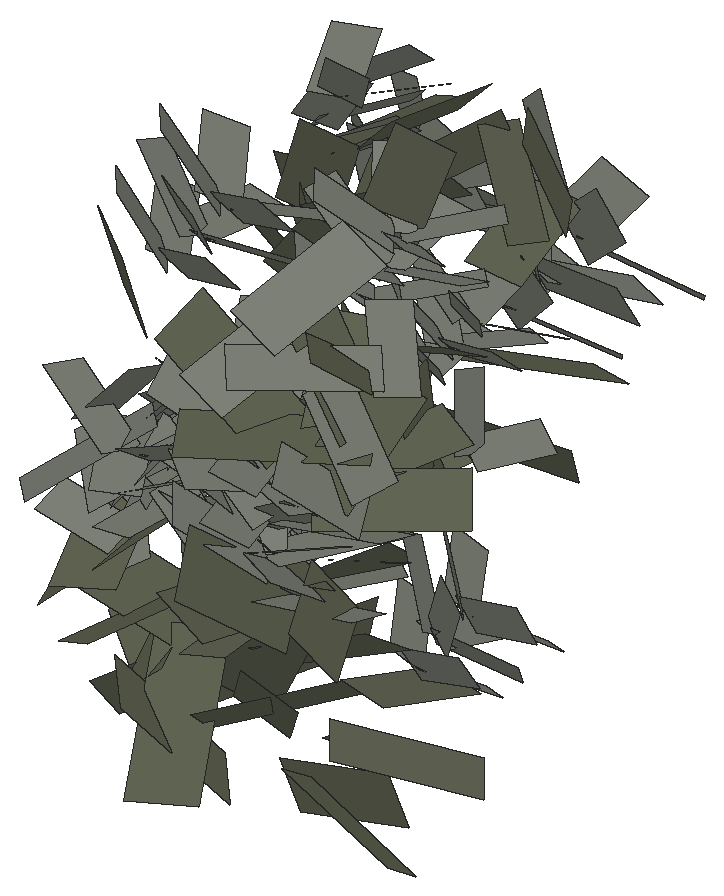
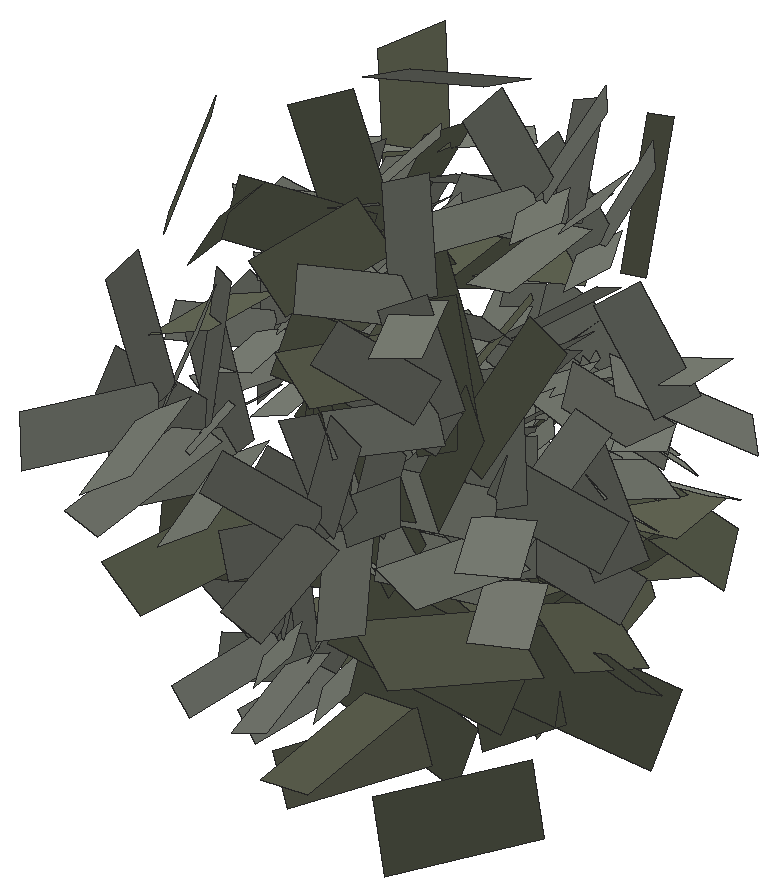
# SketchUp Ruby script. Lengths in inches.
U = 1.inch
M = Sketchup.active_model
def pt(a) = Geom::Point3d.new(a.map { |v| v * U })
def face(e, loops, mat)
  f = e.add_face(loops[0].map { |a| pt(a) })
  loops[1..].each { |l| e.add_face(l.map { |a| pt(a) }).erase! }
  f.material = f.back_material = mat if mat
  f
end
# faces: each face lists its corners as indices into pts; further lists are holes
def faces(e, pts, list, mat = nil) = list.each { |f| face(e, (f[0].is_a?(Array) ? f : [f]).map { |l| l.map { |i| pts[i] } }, mat) }
# xy, xz, yz: faces in a plane at the given z, y or x. An outline is a flat list of corners, or four numbers for a rectangle; further outlines are holes
def ring(l) = l.size == 4 ? [[l[0], l[1]], [l[2], l[1]], [l[2], l[3]], [l[0], l[3]]] : l.each_slice(2).to_a
def flat(e, list, mat, &to3) = list.each { |f| face(e, (f[0].is_a?(Array) ? f : [f]).map { |l| ring(l).map { |u, v| to3.(u, v) } }, mat) }
def xy(e, z, list, mat = nil) = flat(e, list, mat) { |x, y| [x, y, z] }
def xz(e, y, list, mat = nil) = flat(e, list, mat) { |x, z| [x, y, z] }
def yz(e, x, list, mat = nil) = flat(e, list, mat) { |y, z| [x, y, z] }
def lines(e, pts, list) = list.each { |a, b| e.add_line(pt(pts[a]), pt(pts[b])) }
# prism: a flat outline (further loops are holes) pulled along v
def prism(e, loops, v, mat = nil)
  f = face(e, loops, mat); d = Geom::Vector3d.new(v.map { |x| x * U })
  f.pushpull(f.normal.samedirection?(d) ? d.length : -d.length)
end
def box(e, o, s, mat = nil) = prism(e, [[o, [o[0] + s[0], o[1], o[2]], [o[0] + s[0], o[1] + s[1], o[2]], [o[0], o[1] + s[1], o[2]]]], [0, 0, s[2]], mat)
def at(x, y, z, deg = 0) = Geom::Transformation.translation(pt([x, y, z])) * Geom::Transformation.rotation(ORIGIN, Z_AXIS, deg.degrees)
def axes(o, x, y, z) = Geom::Transformation.new([*x, 0, *y, 0, *z, 0, *pt(o).to_a, 1])
def part(name) = M.definitions.add(name)
# library, detail: a bought-in or finely detailed component or shape, given as its bounding box
def library(name, o, s) = part(name).tap { |d| box(d.entities, o, s) }
def detail(e, o, s) = box(e.add_group.entities, o, s)
def put(e, d, t, mat = nil) = e.add_instance(d, t).tap { |i| i.material = mat if mat }
def group(e, t, mat = nil) = e.add_group.tap { |g| g.transformation = t; g.material = mat if mat }.entities
root = M.entities
M.materials.add("viburnumblaasdfas0df1w06d").color = [98, 102, 84]
M.materials.add("viburnumbladsadfasdfad0w122").color = [125, 129, 119]
c1 = part("Component\#315")
p = [[0.25,0,0],[2.05,0.01,0.35],[1.81,4.2,1.66],[0,4.19,1.3125]]
faces(c1.entities,p,[[0,1,2,3]],"viburnumbladsadfasdfad0w122")
c2 = part("viburnumblad2")
put(c2.entities,c1,axes([-19.23,-4.49,-32.18],[83.35428,0,0],[0,79.38502,0],[0,0,83.35428]))
c3 = part("Component\#314")
p = [[0.14,0,0],[2.58,0.05,0.25],[2.44,5.11,2.64],[0,5.05,2.39]]
faces(c3.entities,p,[[0,1,2,3]],"viburnumblaasdfas0df1w06d")
c4 = part("viburnumblad1\#2")
put(c4.entities,c3,axes([-37.25,6.23,19.31],[75.98784,0,0],[0,65.50676,0],[0,0,75.98784]))
put(root,c2,axes([1226.95,207.14,17.86],[0.01077,-0.01075,-0.00083],[0.01118,0.01095,0.00335],[-0.00168,-0.00283,0.01488]))
put(root,c4,axes([1239.8125,210.73,25.15],[-0.01089,-0.0066,0.00527],[0.00777,-0.0139,-0.00135],[0.00514,0.00164,0.01268]))
put(root,c2,axes([1231.69,209.11,19.34],[-0.00239,-0.01136,0.0048],[0.01232,-0.002,0.0014],[-0.0005,0.00498,0.01153]))
put(root,c2,axes([1236.75,207.28,26.68],[0.00842,-0.01125,-0.00685],[0.01063,0.01127,-0.00543],[0.00843,-0.00165,0.01307]))
put(root,c4,axes([1238.97,211.42,14.45],[-0.00936,-0.00465,0.0096],[0.00338,-0.01554,-0.00424],[0.01026,-0.00044,0.00979]))
put(root,c2,axes([1241.4,209.16,19.2],[-0.00545,0.00916,0.00529],[-0.00808,-0.00821,0.00589],[0.00818,-0.00089,0.00998]))
put(root,c4,axes([1236.82,210.48,12.36],[-0.00461,0.01011,0.01059],[-0.01024,-0.0125,0.00748],[0.01168,-0.00415,0.00905]))
put(root,c2,axes([1230.61,207.5,15.64],[0.00178,0.0105,0.00298],[-0.0098,0.00211,-0.00159],[-0.00226,-0.0026,0.01051]))
put(root,c4,axes([1230.86,209.27,23.78],[-0.01166,0.00571,0.00452],[-0.00151,-0.01177,0.01017],[0.0071,0.00732,0.00793]))
put(root,c2,axes([1237.0625,209.16,16.01],[-0.00958,0.01044,0.00206],[-0.00856,-0.00879,0.00474],[0.00514,0.00211,0.0132]))
put(root,c4,axes([1233.03,206.34,5.98],[0.01503,0.00487,0.00033],[-0.00521,0.01551,0.00826],[0.00191,-0.00687,0.0141]))
put(root,c2,axes([1236.97,210.84,15.95],[-0.00988,-0.00976,0.00351],[0.01049,-0.01076,-0.00039],[0.00277,0.00219,0.01388]))
put(root,c2,axes([1230.9,207.19,20.19],[0.00239,0.01136,-0.0048],[-0.01208,0.00314,0.00143],[0.00249,0.00434,0.01152]))
put(root,c2,axes([1236.56,210.93,20.37],[-0.01175,-0.00377,0.00233],[0.00341,-0.01191,-0.00208],[0.00284,-0.00132,0.01217]))
put(root,c4,axes([1229.6,206.2,11.54],[0.01155,-0.00606,0.00446],[0.00831,0.01316,-0.00362],[-0.00229,0.00493,0.01266]))
put(root,c4,axes([1233.6,207.74,21.8],[0.00835,-0.01477,-0.00252],[0.01522,0.00998,-0.00805],[0.00724,0.00145,0.01548]))
put(root,c4,axes([1234.6,209.79,5.19],[-0.01033,0.0106,0.00208],[-0.0106,-0.01173,0.00714],[0.00578,0.00298,0.01347]))
put(root,c4,axes([1227.57,208.05,12.29],[0.0081,-0.01447,0.00211],[0.01627,0.00971,0.00411],[-0.00412,0.00005,0.0162]))
put(root,c4,axes([1229.8,205.78,14.06],[0.01294,0.00473,-0.00003],[-0.00539,0.01473,-0.00308],[-0.00088,0.0025,0.01352]))
put(root,c2,axes([1230.54,208.45,17.9375],[0.007,-0.00987,0.00339],[0.00957,0.00618,-0.0018],[-0.00027,0.0039,0.01194]))
put(root,c2,axes([1235.37,206.35,25.32],[0.01184,-0.00027,-0.00922],[0.00172,0.01671,0.00172],[0.00948,-0.00223,0.01224]))
put(root,c2,axes([1237.53,206.63,28.62],[0.01234,-0.00028,-0.00961],[0.00159,0.01547,0.00159],[0.00948,-0.00223,0.01224]))
put(root,c4,axes([1234.72,212.03,12.13],[-0.01223,0.00026,0.00635],[-0.0009,-0.01592,-0.0011],[0.0063,-0.0012,0.0122]))
put(root,c4,axes([1237.41,209.01,20.64],[0.00084,0.01421,0.00442],[-0.01582,-0.0012,0.00687],[0.00595,-0.00438,0.01294]))
put(root,c2,axes([1229.92,209.05,17.31],[0.00604,-0.00926,0.00001],[0.00806,0.00526,0.00544],[-0.00456,-0.00296,0.00963]))
put(root,c2,axes([1228.79,210.32,19.83],[-0.00259,-0.01229,0.00001],[0.0107,-0.00225,0.00618],[-0.00604,0.00128,0.01094]))
put(root,c2,axes([1230.2,207.53,16.75],[0.01283,-0.0027,-0.00001],[0.00224,0.01066,-0.00301],[0.0007,0.00327,0.01211]))
put(root,c2,axes([1236.01,210.61,18.7],[-0.01046,0.00558,0.00416],[-0.00525,-0.01025,0.00054],[0.00396,-0.00141,0.01184]))
put(root,c2,axes([1235.65,211.38,17.42],[-0.01227,-0.00394,0.00243],[0.00307,-0.01072,-0.00188],[0.00284,-0.00132,0.01217]))
put(root,c2,axes([1235.74,210.03,17.37],[-0.00945,0.00658,-0.00199],[-0.00667,-0.00798,0.00533],[0.00164,0.00544,0.01021]))
put(root,c2,axes([1230.37,207.1,18.52],[0.01038,0.0062,-0.0034],[-0.00717,0.01088,-0.00204],[0.00185,0.00346,0.01194]))
put(root,c2,axes([1241.5,208.6,20.85],[0.00288,0.01252,0.00147],[-0.00904,0.00098,0.00938],[0.00888,-0.00309,0.00888]))
put(root,c2,axes([1229.48,207.8,16.87],[0.00856,0.00558,0.00422],[-0.00642,0.00891,0.00123],[-0.00278,-0.00341,0.01014]))
put(root,c4,axes([1237.26,210.58,6.97],[0.00066,-0.01186,0.00699],[0.01121,-0.00532,-0.01007],[0.0098,0.00532,0.0081]))
put(root,c2,axes([1236.1,211.13,18.5],[-0.01151,-0.00142,0.00146],[0.00195,-0.0101,0.00555],[0.00059,0.0057,0.01018]))
put(root,c2,axes([1235.61,208.65,14.84],[-0.00037,0.01298,-0.00224],[-0.01317,0.00059,0.00559],[0.0056,0.0024,0.01296]))
put(root,c2,axes([1235.57,209.6875,20.35],[-0.00304,0.01166,0.00355],[-0.01127,-0.00408,0.00376],[0.00464,-0.00228,0.01145]))
put(root,c4,axes([1234.08,208.98,8.375],[0.00317,-0.01127,0.00742],[0.01555,0.00409,-0.00043],[-0.00159,0.00725,0.0117]))
put(root,c2,axes([1230.28,208.26,14.39],[0.0081,0.00545,0.00286],[-0.00642,0.00891,0.00123],[-0.00184,-0.00279,0.01054]))
put(root,c4,axes([1240.42,209.32,22.41],[0.00107,0.01287,0.00071],[-0.01171,0.00034,0.00907],[0.0079,-0.00141,0.00892]))
put(root,c2,axes([1235.64,210.98,14.51],[-0.0002,-0.01371,0.00098],[0.01527,-0.0004,-0.00242],[0.00226,0.00098,0.01411]))
put(root,c4,axes([1235.23,211.95,7.27],[-0.01191,-0.00399,0.00577],[0.00688,-0.0137,0.00471],[0.00376,0.00597,0.01189]))
put(root,c2,axes([1235.0625,209.35,16.13],[-0.00179,0.01029,-0.00409],[-0.01223,-0.00094,0.00298],[0.00221,0.00457,0.01052]))
put(root,c2,axes([1235.72,211.41,16.8],[-0.00682,-0.00858,0.00405],[0.00958,-0.00605,0.00332],[-0.00034,0.0052,0.01046]))
put(root,c2,axes([1236.49,209,18.14],[0.00021,0.01428,-0.00102],[-0.01317,0.00059,0.00559],[0.00561,0.00086,0.01315]))
put(root,c4,axes([1238.84,208.55,20.49],[0.01029,0.00428,-0.00658],[0.00078,0.01194,0.00879],[0.00737,-0.00649,0.00685]))
put(root,c2,axes([1235.54,211.9375,19.16],[-0.00616,-0.01091,-0.00086],[0.01132,-0.00616,-0.00282],[0.00193,-0.00206,0.01224]))
put(root,c2,axes([1229.75,208.8,15.67],[0.01032,-0.0026,0.00299],[0.00135,0.01024,0.00424],[-0.00373,-0.00356,0.00978]))
put(root,c4,axes([1233.08,211.32,9.65],[-0.00358,0.0126,0.00711],[-0.01496,-0.00708,0.005],[0.00656,-0.00511,0.01237]))
put(root,c4,axes([1234.71,212.67,14.61],[-0.00859,-0.01039,0.00287],[0.01161,-0.0105,-0.00325],[0.004,0.00034,0.01318]))
put(root,c2,axes([1234.88,210.27,17.48],[-0.00324,0.01089,0.00211],[-0.01127,-0.00408,0.00376],[0.00428,-0.00101,0.01177]))
put(root,c2,axes([1231.44,211.86,25.56],[-0.00734,-0.00647,0.00686],[0.01022,-0.00834,0.00267],[0.00284,0.00722,0.00872]))
put(root,c2,axes([1230.25,208.55,19.69],[0.01229,-0.00259,-0.00001],[0.00249,0.01185,-0.00335],[0.0007,0.00327,0.01211]))
put(root,c2,axes([1231.46,210.52,26.4],[-0.00945,0.00892,-0.00145],[-0.0064,-0.00533,0.00736],[0.00487,0.007,0.00802]))
put(root,c2,axes([1236.94,211.5,17.84],[-0.00021,-0.01428,0.00102],[0.01414,-0.00037,-0.00224],[0.00226,0.00098,0.01411]))
put(root,c2,axes([1232.37,211.98,26.84],[-0.01181,0.00128,0.00407],[0.00154,-0.01046,0.00743],[0.00382,0.0075,0.00815]))
put(root,c2,axes([1228.44,210.26,17.97],[0.0062,-0.01038,0.0034],[0.00931,0.00714,0.00482],[-0.00586,0.00014,0.01111]))
put(root,c2,axes([1234.8,211.15,15.55],[0.00176,-0.01022,0.00282],[0.01152,0.00195,-0.00013],[-0.00039,0.00304,0.01127]))
put(root,c2,axes([1235.05,210.2,18.96],[-0.00186,0.01072,-0.00426],[-0.01132,-0.00087,0.00276],[0.00221,0.00457,0.01052]))
put(root,c4,axes([1232.05,209.32,7.57],[0.00865,0.00658,0.00734],[-0.00992,0.01145,0.00143],[-0.0049,-0.0056,0.0108]))
put(root,c2,axes([1228.44,209.39,16.52],[0.01089,-0.00213,0.00325],[0.002,0.01232,0.0014],[-0.00372,-0.00076,0.01198]))
put(root,c4,axes([1233.8,208.63,13.37],[0.00989,0.00806,-0.00127],[-0.00946,0.01134,-0.00169],[0.00005,0.00193,0.01267]))
put(root,c2,axes([1235.39,211.86,20.9],[0.00304,-0.01166,-0.00355],[0.01206,0.00341,-0.00087],[0.00178,-0.0032,0.01202]))
put(root,c2,axes([1234.36,210.07,19.07],[0.00616,0.01091,0.00086],[-0.01009,0.00525,0.00563],[0.00448,-0.00342,0.01123]))
put(root,c2,axes([1241.47,209.95,24.9],[0.0051,0.01038,-0.00415],[-0.00729,0.00572,0.00502],[0.00694,0.00038,0.0084]))
put(root,c2,axes([1235.13,209.24,16.61],[0.00988,0.00976,-0.00351],[-0.00912,0.01058,0.00376],[0.00511,-0.00035,0.01338]))
put(root,c4,axes([1230.71,208.82,8.77],[0.01224,-0.00166,0.00834],[0.00122,0.01717,0.00163],[-0.00844,-0.00056,0.01227]))
put(root,c4,axes([1237.57,210.72,19.44],[0.00626,-0.00918,-0.00848],[0.01094,0.01129,-0.00412],[0.00772,-0.00395,0.00939]))
put(root,c2,axes([1235.2,212.26,12.91],[-0.0083,0.00785,-0.00197],[-0.00857,-0.00783,0.00492],[0.002,0.00498,0.01141]))
put(root,c4,axes([1233.21,208.9375,11.08],[0.01241,-0.00186,0.00262],[0.00291,0.01409,-0.00376],[-0.00201,0.00365,0.01212]))
put(root,c4,axes([1238.27,210.68,9.32],[0.00753,-0.01126,-0.00255],[0.00884,0.00827,-0.01044],[0.00867,0.00351,0.01012]))
put(root,c2,axes([1235.36,213.53,12.46],[-0.00925,-0.00862,0.00362],[0.00803,-0.00772,0.00213],[0.00081,0.00412,0.01188]))
put(root,c2,axes([1234.42,209.96,17.47],[0.00682,0.00858,-0.00405],[-0.00975,0.00742,-0.00069],[0.00196,0.0036,0.01094]))
put(root,c4,axes([1238.36,209.56,21.39],[0.00971,0.0077,-0.00377],[-0.00736,0.01191,0.00523],[0.00557,-0.00177,0.01033]))
put(root,c4,axes([1228.48,210.5625,6.375],[0.00095,-0.01143,0.01095],[0.01752,0.00456,0.00324],[-0.00472,0.01026,0.01113]))
put(root,c2,axes([1235.07,212.13,18.16],[0.00186,-0.01072,0.00426],[0.01152,0.00195,-0.00013],[-0.00059,0.00423,0.01088]))
put(root,c2,axes([1232.67,212.05,28.52],[-0.00905,0.00854,-0.00139],[-0.00711,-0.00593,0.00818],[0.00487,0.007,0.00802]))
put(root,c2,axes([1235.43,211.04,16.41],[0.00958,-0.01044,-0.00206],[0.01029,0.0098,-0.00181],[0.00273,-0.00027,0.01406]))
put(root,c2,axes([1235.79,213.48,13.95],[-0.01246,0.00054,0.00182],[0.00014,-0.01079,0.00417],[0.00189,0.00451,0.01162]))
put(root,c2,axes([1232.8,213.37,27.68],[-0.00765,-0.00673,0.00714],[0.00947,-0.00772,0.00247],[0.00284,0.00722,0.00872]))
put(root,c2,axes([1234.38,212.22,17.92],[0.00292,-0.01119,-0.00341],[0.01302,0.00368,-0.00094],[0.00178,-0.0032,0.01202]))
put(root,c4,axes([1232.87,213.8125,6.53],[-0.01405,-0.00766,0.00571],[0.01107,-0.01374,0.00878],[0.00057,0.00947,0.0141]))
put(root,c2,axes([1233.9375,210.29,15.875],[0.01201,0.00148,-0.00152],[-0.00157,0.01006,-0.00263],[0.00104,0.00309,0.01122]))
put(root,c2,axes([1234.1,211.2,16.97],[0.00945,-0.00658,0.00199],[0.00631,0.00831,-0.00248],[-0.00002,0.00335,0.01119]))
put(root,c2,axes([1231.55,211.11,27.68],[-0.00099,0.0108,-0.00603],[-0.01031,0.00186,0.00471],[0.00538,0.00602,0.00839]))
put(root,c4,axes([1235.24,212.59,4.09],[-0.00376,-0.0039,0.01194],[0.01323,-0.00731,0.00178],[0.00528,0.01082,0.0052]))
put(root,c4,axes([1236.1,213.6,18.02],[-0.00832,0.00937,0.00389],[-0.0091,-0.01059,0.00604],[0.00643,0.00098,0.01139]))
put(root,c2,axes([1231.43,213.02,26.63],[0.00099,-0.0108,0.00603],[0.0122,-0.00051,-0.00294],[0.0025,0.00634,0.00938]))
put(root,c2,axes([1235.53,213.02,15.8125],[-0.00876,0.00902,-0.0009],[-0.00857,-0.00783,0.00492],[0.00296,0.00403,0.01157]))
put(root,c2,axes([1234.4,210.62,20.88],[0.01175,0.00377,-0.00233],[-0.00262,0.01124,0.00497],[0.00358,-0.00416,0.0113]))
put(root,c4,axes([1234.46,213.24,9.36],[-0.00313,-0.01186,0.00638],[0.01559,-0.00367,0.00082],[0.00085,0.00636,0.01225]))
put(root,c2,axes([1235.8125,214.53,15.39],[-0.00886,-0.00826,0.00347],[0.00892,-0.00858,0.00237],[0.00081,0.00412,0.01188]))
put(root,c2,axes([1235.51,210.51,18.32],[0.01376,-0.00048,-0.00394],[0.00069,0.01429,0.00066],[0.00391,-0.00082,0.01375]))
put(root,c2,axes([1234.2,211.62,19.48],[0.01046,-0.00558,-0.00416],[0.00651,0.0105,0.0023],[0.00246,-0.00407,0.01163]))
put(root,c2,axes([1230.21,210.85,26.82],[0.00649,0.00565,-0.00743],[-0.0085,0.00924,-0.00029],[0.00584,0.00584,0.00823]))
put(root,c4,axes([1236.96,210.8125,19.46],[0.01206,-0.00628,-0.00336],[0.00668,0.01448,-0.00311],[0.00388,0.00091,0.01211]))
put(root,c2,axes([1234.02,211.2,18.62],[0.01151,0.00142,-0.00146],[-0.00175,0.01118,-0.00292],[0.00104,0.00309,0.01122]))
put(root,c4,axes([1236.94,215.24,19.97],[-0.01002,-0.00367,0.00577],[0.0058,-0.01266,0.00203],[0.00466,0.00382,0.01053]))
put(root,c2,axes([1234.54,212.33,14.47],[0.00007,0.01222,-0.00309],[-0.01226,0.00091,0.00331],[0.0034,0.00296,0.01177]))
put(root,c2,axes([1228.05,214.8,15.65],[-0.00906,-0.00899,0.00397],[0.00943,-0.00624,0.00738],[-0.00308,0.00772,0.01046]))
put(root,c2,axes([1234.68,214.47,13.89],[-0.00007,-0.01222,0.00309],[0.01323,-0.00017,-0.00035],[0.00036,0.00309,0.01221]))
put(root,c2,axes([1227.36,214.29,14.07],[0.00073,-0.01105,0.00534],[0.01289,0.00219,0.00278],[-0.00345,0.00543,0.01171]))
put(root,c2,axes([1230.29,212.33,27.51],[0.01181,-0.00128,-0.00407],[-0.00051,0.0116,-0.00495],[0.00406,0.00486,0.00962]))
put(root,c2,axes([1237.46,214.92,24.89],[-0.00706,0.00732,-0.0001],[-0.00736,-0.00703,0.00431],[0.00303,0.00306,0.01018]))
put(root,c2,axes([1238.125,215.85,25.85],[-0.01066,0.00071,0.00285],[0.00002,-0.00983,0.00251],[0.00294,0.00264,0.01033]))
put(root,c2,axes([1237.61,216.07,24.61],[-0.00812,-0.00757,0.00318],[0.00684,-0.00722,0.00028],[0.00201,0.00231,0.01062]))
put(root,c2,axes([1231.62,216.53,15.27],[-0.01116,-0.00699,0.00046],[0.007,-0.01076,0.00634],[-0.00299,0.00562,0.01283]))
put(root,c2,axes([1231.625,216.11,17.15],[-0.01381,0.0032,-0.00202],[-0.0038,-0.01243,0.00635],[-0.00034,0.00659,0.01271]))
put(root,c2,axes([1231.18,212.44,28.89],[0.00765,0.00673,-0.00714],[-0.0085,0.00924,-0.00029],[0.00504,0.00514,0.00906]))
put(root,c2,axes([1231.3125,213.76,28.06],[0.00905,-0.00854,0.00139],[0.00807,0.00744,-0.006],[0.00301,0.00536,0.00976]))
put(root,c2,axes([1233.77,213.72,12.62],[0.00841,-0.00866,0.00086],[0.00975,0.00926,-0.00213],[0.0008,0.00201,0.01242]))
put(root,c2,axes([1238.05,215.26,27.45],[-0.0073,0.00825,0.00099],[-0.00736,-0.00703,0.00431],[0.00384,0.00219,0.01013]))
put(root,c2,axes([1238.32,216.61,27.2],[-0.00778,-0.00725,0.00304],[0.0076,-0.00802,0.00031],[0.00201,0.00231,0.01062]))
put(root,c4,axes([1239.28,214.66,17.94],[-0.00255,0.011,0.00125],[-0.00551,-0.00279,0.01135],[0.00975,0.00148,0.00412]))
put(root,c4,axes([1236.53,216.17,21.99],[-0.00267,-0.01088,0.00464],[0.01349,-0.00382,-0.00119],[0.00218,0.00422,0.01116]))
put(root,c4,axes([1237.78,215.67,19.57],[-0.00734,0.00868,0.00063],[-0.0075,-0.00708,0.00798],[0.0058,0.00404,0.00785]))
put(root,c2,axes([1233.98,213.35,15.97],[0.00886,0.00826,-0.00347],[-0.00846,0.00932,0.00058],[0.00295,0.00192,0.0121]))
put(root,c2,axes([1231.36,217.62,18.51],[-0.01238,-0.00695,0.00189],[0.007,-0.01076,0.00634],[-0.00166,0.00641,0.0127]))
put(root,c2,axes([1233.6,213.63,14.29],[0.01246,-0.00054,-0.00182],[0.00031,0.0125,-0.00159],[0.00187,0.00153,0.01237]))
put(root,c2,axes([1226.97,215.85,16.83],[0.00041,-0.01136,0.00703],[0.01289,0.00219,0.00278],[-0.00352,0.00669,0.01102]))
put(root,c2,axes([1234.26,214.86,15.55],[0.00876,-0.00902,0.0009],[0.00903,0.00857,-0.00197],[0.0008,0.00201,0.01242]))
put(root,c2,axes([1237.03,214.83,26.3125],[0.00034,0.01095,-0.00145],[-0.01033,0.00087,0.00416],[0.0042,0.00122,0.01016]))
put(root,c4,axes([1235.03,214.49,5.98],[0.00779,-0.00697,0.00615],[0.01029,0.00367,-0.00887],[0.00279,0.00941,0.00713]))
put(root,c4,axes([1236.35,214.53,18.68],[0.00125,0.01083,-0.00332],[-0.01199,0.00283,0.0046],[0.00457,0.00236,0.00909]))
put(root,c2,axes([1237.2,216.75,26.01],[-0.00034,-0.01095,0.00145],[0.01148,-0.00057,-0.00162],[0.0016,0.00139,0.01085]))
put(root,c2,axes([1238.21,217.03,8.81],[-0.00478,-0.00491,0.00751],[0.00915,-0.00588,0.00198],[0.00339,0.00769,0.00718]))
put(root,c4,axes([1237.28,214.21,17.88],[0.00373,0.00907,-0.00579],[-0.00694,0.00792,0.00773],[0.00862,0.00055,0.00603]))
put(root,c2,axes([1238.69,217.61,21.06],[-0.00905,-0.00157,0.00381],[0.00376,-0.00932,0.00479],[0.00255,0.00548,0.00745]))
put(root,c4,axes([1231.03,215.5,8.96],[0.00205,-0.01309,0.00844],[0.0176,0.00417,0.0022],[-0.00351,0.00791,0.01312]))
put(root,c2,axes([1239.2,217.27,9.89],[-0.00948,0.00167,0.00544],[0.00331,-0.00711,0.00795],[0.00466,0.00836,0.00554]))
put(root,c4,axes([1237.07,216.69,25.73],[-0.01099,-0.00588,0.00409],[0.00754,-0.00587,0.01184],[-0.00299,0.01058,0.00715]))
put(root,c2,axes([1230.62,217.71,16.4375],[-0.0037,-0.01302,0.00469],[0.0125,-0.00235,0.00334],[-0.00247,0.0054,0.01303]))
put(root,c2,axes([1240.85,215.58,19.58],[-0.00065,0.00993,-0.00423],[-0.00522,0.0028,0.00703],[0.00831,0.00266,0.0042]))
put(root,c4,axes([1233.91,217.66,14.11],[-0.01053,-0.00014,0.0139],[0.01206,-0.01352,0.00899],[0.00923,0.01297,0.00712]))
put(root,c2,axes([1239.1,217.55,22.3],[-0.00889,0.00537,0.00033],[-0.00425,-0.00744,0.00652],[0.00347,0.00529,0.00723]))
put(root,c2,axes([1236.25,216.27,24.93],[0.00701,-0.00792,-0.00095],[0.00872,0.00794,-0.00187],[0.00195,0.00042,0.01087]))
put(root,c2,axes([1239.7,218.54,23.05],[-0.00943,-0.00164,0.00397],[0.00349,-0.00863,0.00444],[0.00255,0.00548,0.00745]))
put(root,c4,axes([1234.7,214.44,16.98],[0.01142,0.00359,-0.00296],[-0.00486,0.01317,-0.00274],[0.00185,0.00298,0.01066]))
put(root,c4,axes([1235.14,214.77,16.96],[0.00961,-0.00181,-0.00747],[-0.00022,0.01383,-0.00363],[0.00726,0.00235,0.00826]))
put(root,c2,axes([1238.04,216.71,21.76],[-0.00329,0.00963,-0.00365],[-0.0081,-0.00098,0.00442],[0.00408,0.00455,0.00739]))
put(root,c2,axes([1236.73,215.59,27.77],[0.00778,0.00725,-0.00304],[-0.00689,0.00834,0.00227],[0.00379,0.0003,0.01038]))
put(root,c2,axes([1230.2,217.01,14.89],[0.00747,-0.01197,0.00496],[0.01097,0.00676,-0.00022],[-0.0023,0.00416,0.01351]))
put(root,c4,axes([1231.26,218.79,20.91],[-0.01185,-0.00554,0.00715],[0.01005,-0.01197,0.00738],[0.00259,0.00922,0.01142]))
put(root,c2,axes([1238.84,218.62,21.89],[-0.00444,-0.00768,0.00528],[0.00919,-0.00479,0.00064],[0.00185,0.00501,0.00791]))
put(root,c2,axes([1237.01,216.9375,27.53],[0.0073,-0.00825,-0.00099],[0.00807,0.00735,-0.00173],[0.00195,0.00042,0.01087]))
put(root,c2,axes([1236.26,216.02,26.38],[0.01066,-0.00071,-0.00285],[0.00069,0.01103,-0.00015],[0.00286,-0.00003,0.01068]))
put(root,c4,axes([1235.59,215.17,8.06],[0.01169,-0.00232,-0.00224],[0.00035,0.01065,-0.00919],[0.00321,0.00758,0.00891]))
put(root,c2,axes([1239.42,218.74,10.43],[-0.0048,-0.00448,0.0089],[0.00915,-0.00588,0.00198],[0.00393,0.00822,0.00626]))
put(root,c2,axes([1237.125,217.26,9.24],[0.00898,-0.00714,0.00125],[0.00484,0.00482,-0.00724],[0.0044,0.00684,0.00749]))
put(root,c2,axes([1237.97,218.21,9.7],[0.00269,-0.008,0.00714],[0.0092,-0.00069,-0.00424],[0.00383,0.00759,0.00707]))
put(root,c2,axes([1239.55,217.78,11.4375],[-0.0086,0.00684,-0.0012],[-0.00415,-0.00354,0.00962],[0.00557,0.00793,0.00532]))
put(root,c2,axes([1238.43,216.83,11],[-0.00269,0.008,-0.00714],[-0.00879,0.00257,0.00619],[0.00614,0.00718,0.00574]))
put(root,c2,axes([1229.59,215.375,15.42],[0.01189,0.00667,-0.00181],[-0.00777,0.01295,-0.00333],[0.00008,0.00361,0.01386]))
put(root,c2,axes([1240.4,216.59,19.76],[0.00544,-0.00271,-0.00718],[0.0003,0.00981,-0.00339],[0.00825,0.00152,0.00476]))
put(root,c2,axes([1237.35,216.24,10.1875],[0.00461,0.0043,-0.00854],[-0.00856,0.00831,-0.00043],[0.00603,0.00655,0.00655]))
put(root,c4,axes([1229.8,215.15,5.5],[0.00521,-0.00318,0.0136],[0.01189,0.01244,-0.00164],[-0.00949,0.00985,0.00593]))
put(root,c2,axes([1238.96,217.7,23.71],[-0.00315,0.00923,-0.0035],[-0.009,-0.00109,0.00491],[0.00408,0.00455,0.00739]))
put(root,c4,axes([1229.76,215.41,11.59],[0.01313,-0.00582,0.00636],[0.00841,0.01593,-0.00278],[-0.00467,0.00494,0.01417]))
put(root,c4,axes([1230.42,219.45,21.7],[-0.01202,0.00402,-0.00269],[-0.00561,-0.01134,0.00795],[0.00019,0.00723,0.00942]))
put(root,c2,axes([1238.02,217.27,22.79],[0.00444,0.00768,-0.00528],[-0.00777,0.00538,0.00119],[0.00402,0.0037,0.00783]))
put(root,c2,axes([1229.72,218.3,18.16],[0.00715,-0.01146,0.00475],[0.01219,0.00751,-0.00024],[-0.0023,0.00416,0.01351]))
put(root,c2,axes([1229.23,216.8,16.72],[0.01381,-0.0032,0.00202],[0.00375,0.01421,-0.00318],[-0.00124,0.00342,0.01385]))
put(root,c2,axes([1237.17,217.42,21.79],[0.00829,0.00118,-0.00446],[-0.00277,0.00969,-0.0025],[0.00431,0.00339,0.00782]))
put(root,c2,axes([1238.6875,219.37,22.97],[0.00315,-0.00923,0.0035],[0.00972,0.00216,-0.00297],[0.00178,0.00415,0.00836]))
put(root,c2,axes([1237.5,217.63,10.76],[0.00948,-0.00167,-0.00544],[-0.00216,0.00929,-0.00661],[0.00531,0.00641,0.00728]))
put(root,c2,axes([1228.96,216.75,18.7],[0.01238,0.00695,-0.00189],[-0.0072,0.01199,-0.00308],[0.00008,0.00361,0.01386]))
put(root,c2,axes([1237.59,218.58,22.32],[0.00889,-0.00537,-0.00033],[0.00481,0.00824,-0.00432],[0.00239,0.00342,0.00851]))
put(root,c2,axes([1238.18,219.12,10.96],[0.0086,-0.00684,0.0012],[0.00538,0.00535,-0.00804],[0.0044,0.00684,0.00749]))
put(root,c2,axes([1238.31,218.16,11.96],[0.0048,0.00448,-0.0089],[-0.00793,0.0077,-0.0004],[0.00603,0.00655,0.00655]))
put(root,c4,axes([1235.11,218.29,26.65],[0.00085,-0.00676,0.01003],[0.01236,0.00601,0.00299],[-0.00572,0.00864,0.0063]))
put(root,c2,axes([1231.33,221.84,28.41],[-0.00994,-0.00547,0.00222],[0.00636,-0.00933,0.00551],[-0.00082,0.00596,0.01103]))
put(root,c4,axes([1241.92,220.25,26.98],[-0.00677,0.00906,0.00107],[-0.00671,-0.00636,0.00903],[0.00707,0.00408,0.0069]))
put(root,c2,axes([1237.94,218.53,23.64],[0.00943,0.00164,-0.00397],[-0.00277,0.00969,-0.0025],[0.00332,0.00323,0.0083]))
put(root,c4,axes([1229.72,221.49,22.52],[-0.01137,-0.00525,0.00325],[0.00699,-0.00886,0.00961],[-0.00151,0.00884,0.00798]))
put(root,c4,axes([1240.32,219.15,26.31],[0.00134,0.01062,-0.0039],[-0.01115,0.00362,0.00577],[0.00594,0.00252,0.00833]))
put(root,c4,axes([1230.89,220.22,20.58],[-0.00982,0.00575,-0.00616],[-0.00925,-0.00382,0.01097],[0.00277,0.01054,0.00496]))
put(root,c4,axes([1233.82,220.63,16.09],[0.0041,-0.00986,0.01208],[0.01717,-0.00172,-0.00723],[0.00492,0.01267,0.00868]))
put(root,c4,axes([1230.02,220.53,23.09],[0.00221,-0.01095,0.00807],[0.01572,0.00285,-0.00044],[-0.00114,0.008,0.01116]))
put(root,c4,axes([1233.66,218.75,28.32],[0.00897,-0.0006,0.00814],[0.00562,0.01175,-0.00532],[-0.00657,0.00665,0.00773]))
put(root,c4,axes([1238.4375,219.07,24.83],[0.01113,0.00289,-0.00438],[-0.00454,0.01328,-0.00273],[0.00348,0.00335,0.01016]))
put(root,c2,axes([1237.75,223.41,20.6],[-0.0106,-0.00225,0.00809],[0.00771,-0.01018,0.00728],[0.00487,0.01032,0.00927]))
put(root,c2,axes([1230.07,222.3,28.21],[0.00655,-0.0105,0.00435],[0.00979,0.0053,-0.00197],[-0.0002,0.0047,0.01165]))
put(root,c2,axes([1228.48,223.96,25.5],[-0.00824,-0.00797,0.00286],[0.00803,-0.0057,0.00726],[-0.00361,0.00659,0.00792]))
put(root,c4,axes([1230.96,222.54,20.27],[-0.01249,0.00074,0.00321],[0.00342,-0.00484,0.01344],[0.00175,0.01171,0.00271]))
put(root,c2,axes([1238.65,223.63,22.34],[-0.01262,0.00712,0.00249],[-0.00199,-0.00788,0.01243],[0.00728,0.01023,0.00765]))
put(root,c2,axes([1228.09,223.32,24.22],[-0.00014,-0.00961,0.00594],[0.01198,0.00212,0.00345],[-0.00404,0.00568,0.00838]))
put(root,c2,axes([1229.53,220.94,28.86],[0.01039,0.00506,-0.00344],[-0.00658,0.01149,-0.00298],[0.00188,0.00411,0.01172]))
put(root,c4,axes([1229.23,220.7,25.53],[0.0119,-0.00534,0.00444],[0.00766,0.01326,-0.00459],[-0.00215,0.00555,0.01243]))
put(root,c2,axes([1237.66,225.21,21.4375],[-0.00284,-0.00899,0.01128],[0.01228,-0.00546,-0.00125],[0.00539,0.01,0.00933]))
put(root,c2,axes([1236.38,224.21,20.65],[0.00722,-0.01189,0.00649],[0.01053,0.00219,-0.0077],[0.0056,0.00897,0.01021]))
put(root,c2,axes([1239.36,225.54,22.89],[-0.01093,-0.00132,0.00974],[0.00771,-0.01018,0.00728],[0.00609,0.01052,0.00826]))
put(root,c4,axes([1234.05,221.85,18.83],[0.01385,-0.00786,0.00256],[0.00839,0.01058,-0.01294],[0.00399,0.01072,0.01136]))
put(root,c2,axes([1230.66,224.79,21.88],[-0.01171,0.00153,-0.0034],[-0.00332,-0.0036,0.00923],[0.00008,0.01052,0.00323]))
put(root,c2,axes([1227.69,225.03,26.32],[-0.00014,-0.01001,0.00619],[0.0111,0.00196,0.00319],[-0.00404,0.00568,0.00838]))
put(root,c2,axes([1227.18,223.93,25.22],[0.00804,-0.00619,0.0059],[0.00785,0.00862,-0.00178],[-0.00364,0.00486,0.00899]))
put(root,c2,axes([1230.09,225.39,20.65],[-0.00352,-0.00505,0.00939],[0.01197,-0.00026,0.00408],[-0.00173,0.01006,0.00403]))
put(root,c2,axes([1238.73,224.57,24.35],[-0.00691,0.01139,-0.00621],[-0.01,-0.00019,0.01077],[0.00826,0.00929,0.00783]))
put(root,c2,axes([1235.86,223.12,22.07],[0.01049,0.00127,-0.00935],[-0.00649,0.01342,-0.00547],[0.00778,0.00774,0.00978]))
put(root,c2,axes([1237.14,223.68,23.46],[0.00284,0.00899,-0.01128],[-0.01167,0.00819,0.00358],[0.00847,0.00827,0.00872]))
put(root,c2,axes([1230.6875,226.43,21.54],[-0.01052,-0.00268,0.00462],[0.00552,-0.00368,0.01018],[-0.00102,0.01046,0.0033]))
put(root,c2,axes([1230.36,225.78,22.71],[-0.00534,0.00476,-0.00922],[-0.00963,-0.00133,0.0047],[0.00092,0.0102,0.00386]))
put(root,c2,axes([1236.45,224.96,22.65],[0.01262,-0.00712,-0.00249],[0.00385,0.01054,-0.01059],[0.00659,0.00804,0.0104]))
put(root,c2,axes([1237.85,226.62,22.96],[0.00691,-0.01139,0.00621],[0.0117,0.00243,-0.00856],[0.0056,0.00897,0.01021]))
put(root,c2,axes([1230.77,227.31,22.88],[-0.01122,0.00147,-0.00326],[-0.00368,-0.004,0.01025],[0.00008,0.01052,0.00323]))
put(root,c2,axes([1229.46,226.66,21.09],[0.00534,-0.00476,0.00922],[0.0104,0.00387,-0.00404],[-0.00165,0.00955,0.00498]))
put(root,c2,axes([1228.78,226.02,22.26],[0.01052,0.00268,-0.00462],[-0.0054,0.00599,-0.0087],[0.00028,0.0093,0.00555]))
put(root,c2,axes([1230.33,227.96,21.63],[-0.00367,-0.00526,0.00978],[0.01109,-0.00025,0.00378],[-0.00173,0.01006,0.00403]))
put(root,c2,axes([1237.23,225.65,24.42],[0.01093,0.00132,-0.00974],[-0.00601,0.01242,-0.00506],[0.00778,0.00774,0.00978]))
put(root,c2,axes([1228.91,227.73,22.01],[0.01122,-0.00147,0.00326],[0.00359,0.00643,-0.00917],[-0.00081,0.00924,0.00561]))
